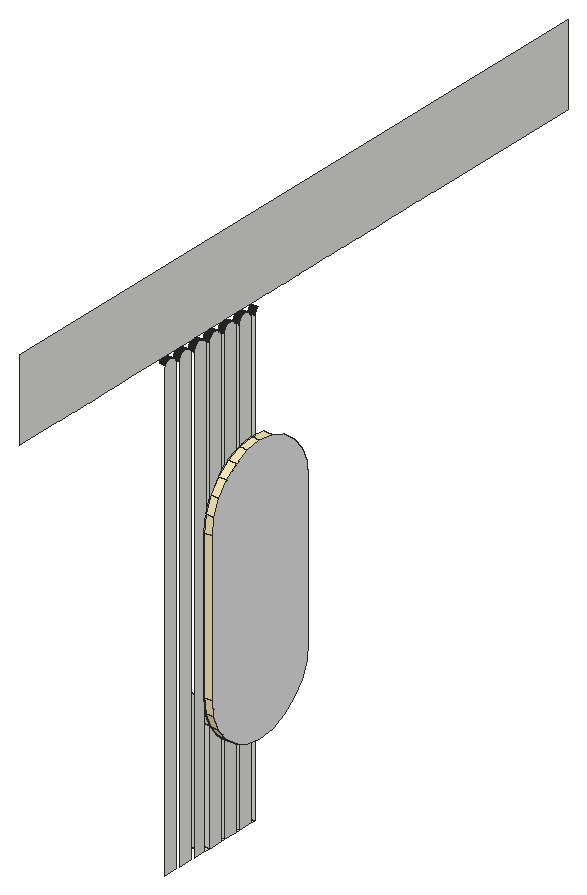
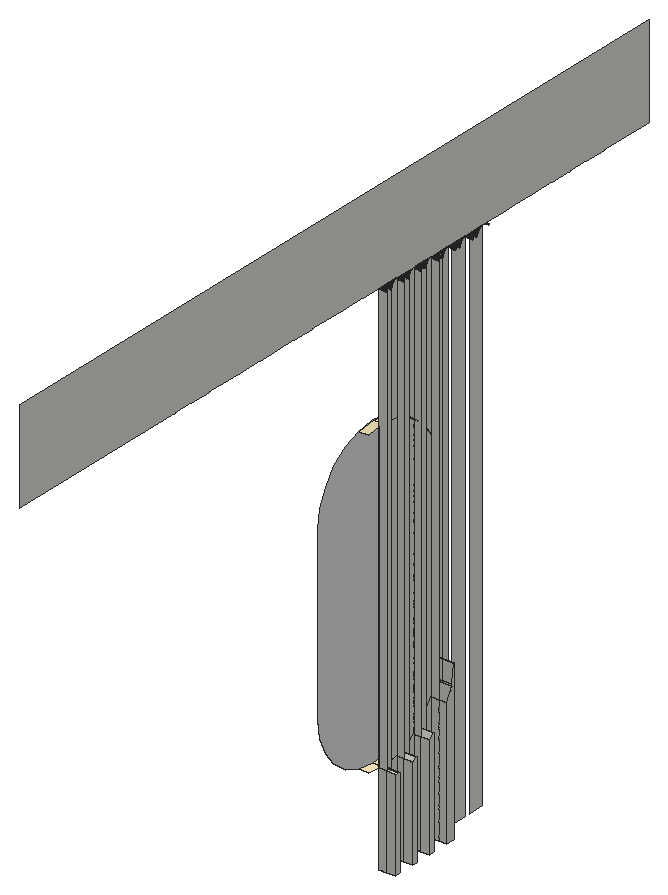
# SketchUp Ruby script. Lengths in inches.
U = 1.inch
M = Sketchup.active_model
def pt(a) = Geom::Point3d.new(a.map { |v| v * U })
def face(e, loops, mat)
  f = e.add_face(loops[0].map { |a| pt(a) })
  loops[1..].each { |l| e.add_face(l.map { |a| pt(a) }).erase! }
  f.material = f.back_material = mat if mat
  f
end
# faces: each face lists its corners as indices into pts; further lists are holes
def faces(e, pts, list, mat = nil) = list.each { |f| face(e, (f[0].is_a?(Array) ? f : [f]).map { |l| l.map { |i| pts[i] } }, mat) }
# xy, xz, yz: faces in a plane at the given z, y or x. An outline is a flat list of corners, or four numbers for a rectangle; further outlines are holes
def ring(l) = l.size == 4 ? [[l[0], l[1]], [l[2], l[1]], [l[2], l[3]], [l[0], l[3]]] : l.each_slice(2).to_a
def flat(e, list, mat, &to3) = list.each { |f| face(e, (f[0].is_a?(Array) ? f : [f]).map { |l| ring(l).map { |u, v| to3.(u, v) } }, mat) }
def xy(e, z, list, mat = nil) = flat(e, list, mat) { |x, y| [x, y, z] }
def xz(e, y, list, mat = nil) = flat(e, list, mat) { |x, z| [x, y, z] }
def yz(e, x, list, mat = nil) = flat(e, list, mat) { |y, z| [x, y, z] }
def lines(e, pts, list) = list.each { |a, b| e.add_line(pt(pts[a]), pt(pts[b])) }
# prism: a flat outline (further loops are holes) pulled along v
def prism(e, loops, v, mat = nil)
  f = face(e, loops, mat); d = Geom::Vector3d.new(v.map { |x| x * U })
  f.pushpull(f.normal.samedirection?(d) ? d.length : -d.length)
end
def box(e, o, s, mat = nil) = prism(e, [[o, [o[0] + s[0], o[1], o[2]], [o[0] + s[0], o[1] + s[1], o[2]], [o[0], o[1] + s[1], o[2]]]], [0, 0, s[2]], mat)
def at(x, y, z, deg = 0) = Geom::Transformation.translation(pt([x, y, z])) * Geom::Transformation.rotation(ORIGIN, Z_AXIS, deg.degrees)
def axes(o, x, y, z) = Geom::Transformation.new([*x, 0, *y, 0, *z, 0, *pt(o).to_a, 1])
def part(name) = M.definitions.add(name)
# library, detail: a bought-in or finely detailed component or shape, given as its bounding box
def library(name, o, s) = part(name).tap { |d| box(d.entities, o, s) }
def detail(e, o, s) = box(e.add_group.entities, o, s)
def put(e, d, t, mat = nil) = e.add_instance(d, t).tap { |i| i.material = mat if mat }
def group(e, t, mat = nil) = e.add_group.tap { |g| g.transformation = t; g.material = mat if mat }.entities
root = M.entities
M.materials.add("Heather_PantShadow").color = [249, 233, 187]
M.materials.add("[Mirror 02]").color = [229, 229, 229]
xy(root,39.466,[[7.875,42.018,10,43.106],[7.875,45.1875,10,45.893],[7.875,47.975,10,48.681],[7.875,50.762,10,51.468]])
xy(root,108,[[9,35.73,10,35.839],[9,38.517,10,38.626],[9,41.305,10,41.414],[9,44.092,10,44.201],[9,46.88,10,46.989],
  [9,49.667,10,49.776]])
xz(root,42.018,[[7.875,39.466,10,60.077]])
xz(root,42.018,[[10,60.077,11.25,82.153]],"Heather_PantShadow")
xz(root,43.106,[[7.875,39.466,9,55.879],[9,39.466,10,55.879],[9,55.879,10,106.961]])
xz(root,45.1875,[[7.875,39.466,9,53.349],[9,39.466,10,53.349],[9,53.349,10,106.961]])
xz(root,45.893,[[7.875,39.466,9,52.807],[9,39.466,10,52.807],[9,52.807,10,106.961]])
xz(root,47.975,[[7.875,39.466,9,51.741],[9,39.466,10,51.741],[9,51.741,10,106.961]])
xz(root,48.681,[[7.875,39.466,9,51.466],[9,39.466,10,51.466],[9,51.466,10,106.961]])
xz(root,50.762,[[7.875,39.466,9,51.192],[9,39.466,10,51.192],[9,51.192,10,106.961]])
xz(root,51.468,[[7.875,39.466,9,51.242],[9,39.466,10,51.242],[9,51.242,10,106.961]])
yz(root,7.875,[[42.018,39.466,43.106,39.466,43.106,55.879,42.4,57.583,42.322,57.772,42.018,60.077],[45.1875,39.466,45.893,39.466,45.893,52.807,45.1875,53.349],[47.975,39.466,48.681,39.466,48.681,51.466,48.62,51.474,47.975,51.741],[50.762,39.466,51.468,39.466,51.468,51.242,50.925,51.17,50.762,51.192]])
yz(root,9,[[9,108,16.217,108,16.272,108.001,16.326,108,19.005,108,19.059,108.001,19.114,108,21.792,108,21.847,108.001,21.901,108,24.58,108,24.634,108.001,24.689,108,27.367,108,27.422,108.001,27.476,108,30.155,108,30.209,108.001,30.264,108,32.942,108,32.997,108.001,33.051,108,35.73,108,35.784,108.001,35.839,108,38.517,108,38.572,108.001,38.626,108,41.305,108,41.359,108.001,41.414,108,44.092,108,44.147,108.001,44.201,108,46.88,108,46.934,108.001,46.989,108,49.667,108,49.722,108.001,49.776,108,52.455,108,52.509,108.001,52.564,108,55.242,108,55.297,108.001,55.351,108,58.03,108,58.084,108.001,58.139,108,60.817,108,60.872,108.001,60.926,108,63.605,108,63.659,108.001,63.714,108,66.392,108,66.447,108.001,66.501,108,69.18,108,69.234,108.001,69.289,108,71.967,108,72.022,108.001,72.076,108,74.755,108,74.809,108.001,74.864,108,77.542,108,77.597,108.001,77.651,108,80.33,108,80.384,108.001,80.439,108,83.117,108,83.172,108.001,83.226,108,85.905,108,85.959,108.001,86.014,108,111,108,111,120,9,120],[35.73,108,35.839,108,35.784,108.001],[38.517,108,38.626,108,38.572,108.001],[41.305,108,41.414,108,41.359,108.001],[44.092,108,44.201,108,44.147,108.001],
  [46.88,108,46.989,108,46.934,108.001],[49.667,108,49.776,108,49.722,108.001]])
yz(root,10,[[34.743,39.466,36.825,39.466,36.825,106.961,36.824,107.015,36.819,107.069,36.812,107.123,36.802,107.177,36.79,107.23,36.774,107.282,36.756,107.334,36.735,107.384,36.712,107.433,36.686,107.481,36.657,107.528,36.626,107.572,36.593,107.616,36.558,107.657,36.52,107.697,36.481,107.734,36.439,107.769,36.396,107.803,36.351,107.834,36.305,107.862,36.257,107.888,36.208,107.911,36.157,107.932,36.106,107.95,36.054,107.966,36.001,107.979,35.947,107.989,35.893,107.996,35.839,108,35.73,108,35.675,107.996,35.621,107.989,35.568,107.979,35.515,107.966,35.463,107.95,35.411,107.932,35.361,107.911,35.312,107.888,35.264,107.862,35.217,107.834,35.173,107.803,35.129,107.769,35.088,107.734,35.048,107.697,35.011,107.657,34.975,107.616,34.942,107.572,34.911,107.528,34.883,107.481,34.857,107.433,34.833,107.384,34.8125,107.334,34.794,107.282,34.779,107.23,34.766,107.177,34.756,107.123,34.749,107.069,34.745,107.015,34.743,106.961],[37.531,39.466,39.612,39.466,39.612,106.961,39.611,107.015,39.607,107.069,39.6,107.123,39.59,107.177,39.577,107.23,39.562,107.282,39.543,107.334,39.523,107.384,39.499,107.433,39.473,107.481,39.445,107.528,39.414,107.572,39.381,107.616,39.345,107.657,39.308,107.697,39.268,107.734,39.227,107.769,39.183,107.803,39.139,107.834,39.092,107.862,39.044,107.888,38.995,107.911,38.945,107.932,38.893,107.95,38.841,107.966,38.788,107.979,38.735,107.989,38.681,107.996,38.626,108,38.517,108,38.463,107.996,38.409,107.989,38.355,107.979,38.302,107.966,38.25,107.95,38.199,107.932,38.148,107.911,38.099,107.888,38.051,107.862,38.005,107.834,37.96,107.803,37.917,107.769,37.875,107.734,37.836,107.697,37.798,107.657,37.763,107.616,37.73,107.572,37.699,107.528,37.67,107.481,37.644,107.433,37.621,107.384,37.6,107.334,37.582,107.282,37.566,107.23,37.554,107.177,37.544,107.123,37.537,107.069,37.532,107.015,37.531,106.961],[40.318,39.466,42.018,39.466,42.018,82.153,42.322,84.458,42.4,84.647,42.4,106.961,42.399,107.015,42.394,107.069,42.387,107.123,42.377,107.177,42.365,107.23,42.349,107.282,42.331,107.334,42.31,107.384,42.287,107.433,42.261,107.481,42.232,107.528,42.201,107.572,42.168,107.616,42.133,107.657,42.095,107.697,42.056,107.734,42.014,107.769,41.971,107.803,41.926,107.834,41.88,107.862,41.832,107.888,41.783,107.911,41.732,107.932,41.681,107.95,41.629,107.966,41.576,107.979,41.522,107.989,41.468,107.996,41.414,108,41.305,108,41.25,107.996,41.196,107.989,41.143,107.979,41.09,107.966,41.038,107.95,40.986,107.932,40.936,107.911,40.887,107.888,40.839,107.862,40.792,107.834,40.748,107.803,40.704,107.769,40.663,107.734,40.623,107.697,40.586,107.657,40.55,107.616,40.517,107.572,40.486,107.528,40.458,107.481,40.432,107.433,40.408,107.384,40.388,107.334,40.369,107.282,40.354,107.23,40.341,107.177,40.331,107.123,40.324,107.069,40.32,107.015,40.318,106.961],[43.106,39.466,45.1875,39.466,45.1875,53.349,44.627,53.779,43.212,55.624,43.106,55.879],[45.893,39.466,47.975,39.466,47.975,51.741,46.472,52.364,45.893,52.807],
  [48.681,39.466,50.762,39.466,50.762,51.192,48.681,51.466],[50.925,51.17,50.762,51.192,50.762,91.038,50.925,91.06,51.468,90.988,51.468,51.242],[50.762,51.192,50.762,91.038,48.681,90.764,48.681,51.466],[48.681,51.466,48.62,51.474,47.975,51.741,47.975,90.489,48.62,90.756,48.681,90.764],[47.975,51.741,47.975,90.489,46.472,89.866,45.893,89.423,45.893,52.807,46.472,52.364],
  [45.893,52.807,45.1875,53.349,45.1875,88.881,45.893,89.423],[45.1875,53.349,45.1875,88.881,44.627,88.451,43.212,86.606,43.106,86.351,43.106,55.879,43.212,55.624,44.627,53.779],[43.106,55.879,42.4,57.583,42.4,84.647,43.106,86.351],[42.4,57.583,42.4,84.647,42.322,84.458,42.018,82.153,42.018,60.077,42.322,57.772],[43.106,86.351,43.212,86.606,44.627,88.451,45.1875,88.881,45.1875,106.961,45.186,107.015,45.182,107.069,45.175,107.123,45.165,107.177,45.152,107.23,45.137,107.282,45.118,107.334,45.098,107.384,45.074,107.433,45.048,107.481,45.02,107.528,44.989,107.572,44.956,107.616,44.92,107.657,44.883,107.697,44.843,107.734,44.802,107.769,44.758,107.803,44.714,107.834,44.667,107.862,44.619,107.888,44.57,107.911,44.52,107.932,44.468,107.95,44.416,107.966,44.363,107.979,44.31,107.989,44.256,107.996,44.201,108,44.092,108,44.038,107.996,43.984,107.989,43.93,107.979,43.877,107.966,43.825,107.95,43.774,107.932,43.723,107.911,43.674,107.888,43.626,107.862,43.58,107.834,43.535,107.803,43.492,107.769,43.45,107.734,43.411,107.697,43.373,107.657,43.338,107.616,43.305,107.572,43.274,107.528,43.245,107.481,43.219,107.433,43.196,107.384,43.175,107.334,43.157,107.282,43.141,107.23,43.129,107.177,43.119,107.123,43.112,107.069,43.107,107.015,43.106,106.961],
  [45.893,89.423,46.472,89.866,47.975,90.489,47.975,106.961,47.974,107.015,47.969,107.069,47.962,107.123,47.952,107.177,47.94,107.23,47.924,107.282,47.906,107.334,47.885,107.384,47.862,107.433,47.836,107.481,47.807,107.528,47.776,107.572,47.743,107.616,47.708,107.657,47.67,107.697,47.631,107.734,47.589,107.769,47.546,107.803,47.501,107.834,47.455,107.862,47.407,107.888,47.358,107.911,47.307,107.932,47.256,107.95,47.204,107.966,47.151,107.979,47.097,107.989,47.043,107.996,46.989,108,46.88,108,46.825,107.996,46.771,107.989,46.718,107.979,46.665,107.966,46.613,107.95,46.561,107.932,46.511,107.911,46.462,107.888,46.414,107.862,46.367,107.834,46.323,107.803,46.279,107.769,46.238,107.734,46.198,107.697,46.161,107.657,46.125,107.616,46.092,107.572,46.061,107.528,46.033,107.481,46.007,107.433,45.983,107.384,45.963,107.334,45.944,107.282,45.929,107.23,45.916,107.177,45.906,107.123,45.899,107.069,45.895,107.015,45.893,106.961],[48.681,90.764,50.762,91.038,50.762,106.961,50.761,107.015,50.757,107.069,50.75,107.123,50.74,107.177,50.727,107.23,50.712,107.282,50.693,107.334,50.673,107.384,50.649,107.433,50.623,107.481,50.595,107.528,50.564,107.572,50.531,107.616,50.495,107.657,50.458,107.697,50.418,107.734,50.377,107.769,50.333,107.803,50.289,107.834,50.242,107.862,50.194,107.888,50.145,107.911,50.095,107.932,50.043,107.95,49.991,107.966,49.938,107.979,49.885,107.989,49.831,107.996,49.776,108,49.667,108,49.613,107.996,49.559,107.989,49.505,107.979,49.452,107.966,49.4,107.95,49.349,107.932,49.298,107.911,49.249,107.888,49.201,107.862,49.155,107.834,49.11,107.803,49.067,107.769,49.025,107.734,48.986,107.697,48.948,107.657,48.913,107.616,48.88,107.572,48.849,107.528,48.82,107.481,48.794,107.433,48.771,107.384,48.75,107.334,48.732,107.282,48.716,107.23,48.704,107.177,48.694,107.123,48.687,107.069,48.682,107.015,48.681,106.961]])
yz(root,11.25,[[50.925,51.17,53.23,51.474,55.378,52.364,57.222,53.779,58.638,55.624,59.528,57.772,59.831,60.077,59.831,82.153,59.528,84.458,58.638,86.606,57.222,88.451,55.378,89.866,53.23,90.756,50.925,91.06,48.62,90.756,46.472,89.866,44.627,88.451,43.212,86.606,42.322,84.458,42.018,82.153,42.018,60.077,42.322,57.772,43.212,55.624,44.627,53.779,46.472,52.364,48.62,51.474]],"[Mirror 02]")
p = [[11.25,50.925,51.17],[11.25,48.62,51.474],[10,48.62,51.474],[10,48.681,51.466],[10,50.762,51.192],[10,50.925,51.17],
  [9,50.762,51.192],[7.875,50.762,51.192],[7.875,50.925,51.17],[10,51.468,51.242],[7.875,51.468,51.242],[9,51.468,51.242],
  [11.25,53.23,51.474],[10,53.23,51.474],[11.25,46.472,52.364],[10,46.472,52.364],[10,47.975,51.741],[9,47.975,51.741],
  [7.875,47.975,51.741],[7.875,48.62,51.474],[7.875,48.681,51.466],[9,48.681,51.466],[11.25,44.627,53.779],[10,44.627,53.779],
  [10,45.1875,53.349],[10,45.893,52.807],[9,45.1875,53.349],[7.875,45.1875,53.349],[7.875,45.893,52.807],[9,45.893,52.807],
  [11.25,43.212,55.624],[10,43.212,55.624],[11.25,42.322,57.772],[10,42.322,57.772],[10,42.4,57.583],[10,43.106,55.879],
  [9,42.4,57.583],[7.875,42.4,57.583],[7.875,43.106,55.879],[9,43.106,55.879],[7.875,42.322,57.772],[10,42.018,60.077],
  [7.875,42.018,60.077],[11.25,42.018,60.077],[11.25,42.018,82.153],[11.25,42.322,84.458],[10,42.322,84.458],[10,42.018,82.153],
  [11.25,43.212,86.606],[10,43.212,86.606],[10,43.106,86.351],[10,42.4,84.647],[11.25,44.627,88.451],[10,44.627,88.451],
  [11.25,46.472,89.866],[10,46.472,89.866],[10,45.893,89.423],[10,45.1875,88.881],[11.25,48.62,90.756],[10,48.62,90.756],
  [10,47.975,90.489],[11.25,50.925,91.06],[10,50.925,91.06],[10,50.762,91.038],[10,48.681,90.764],[11.25,53.23,90.756],
  [10,53.23,90.756],[10,51.468,90.988],[9,36.824,107.015],[9,36.819,107.069],[10,36.819,107.069],[10,36.824,107.015],
  [9,36.825,106.961],[10,36.825,106.961],[9,37.532,107.015],[9,37.531,106.961],[10,37.531,106.961],[10,37.532,107.015],
  [9,37.537,107.069],[10,37.537,107.069],[9,39.611,107.015],[9,39.607,107.069],[10,39.607,107.069],[10,39.611,107.015],
  [9,39.612,106.961],[10,39.612,106.961],[9,40.32,107.015],[9,40.318,106.961],[10,40.318,106.961],[10,40.32,107.015],
  [9,40.324,107.069],[10,40.324,107.069],[9,42.399,107.015],[9,42.394,107.069],[10,42.394,107.069],[10,42.399,107.015],
  [9,42.4,106.961],[10,42.4,106.961],[9,43.107,107.015],[9,43.106,106.961],[10,43.106,106.961],[10,43.107,107.015],
  [9,43.112,107.069],[10,43.112,107.069],[9,45.186,107.015],[9,45.182,107.069],[10,45.182,107.069],[10,45.186,107.015],
  [9,45.1875,106.961],[10,45.1875,106.961],[9,45.895,107.015],[9,45.893,106.961],[10,45.893,106.961],[10,45.895,107.015],
  [9,45.899,107.069],[10,45.899,107.069],[9,47.974,107.015],[9,47.969,107.069],[10,47.969,107.069],[10,47.974,107.015],
  [9,47.975,106.961],[10,47.975,106.961],[9,48.682,107.015],[9,48.681,106.961],[10,48.681,106.961],[10,48.682,107.015],
  [9,48.687,107.069],[10,48.687,107.069],[9,50.761,107.015],[9,50.757,107.069],[10,50.757,107.069],[10,50.761,107.015],
  [9,50.762,106.961],[10,50.762,106.961],[9,51.47,107.015],[9,51.468,106.961],[10,51.468,106.961],[10,51.47,107.015],
  [9,51.474,107.069],[10,51.474,107.069],[9,36.812,107.123],[9,36.802,107.177],[10,36.802,107.177],[10,36.812,107.123],
  [9,37.544,107.123],[10,37.544,107.123],[9,37.554,107.177],[10,37.554,107.177],[9,39.6,107.123],[9,39.59,107.177],
  [10,39.59,107.177],[10,39.6,107.123],[9,40.331,107.123],[10,40.331,107.123],[9,40.341,107.177],[10,40.341,107.177],
  [9,42.387,107.123],[9,42.377,107.177],[10,42.377,107.177],[10,42.387,107.123],[9,43.119,107.123],[10,43.119,107.123],
  [9,43.129,107.177],[10,43.129,107.177],[9,45.175,107.123],[9,45.165,107.177],[10,45.165,107.177],[10,45.175,107.123],
  [9,45.906,107.123],[10,45.906,107.123],[9,45.916,107.177],[10,45.916,107.177],[9,47.962,107.123],[9,47.952,107.177],
  [10,47.952,107.177],[10,47.962,107.123],[9,48.694,107.123],[10,48.694,107.123],[9,48.704,107.177],[10,48.704,107.177],
  [9,50.75,107.123],[9,50.74,107.177],[10,50.74,107.177],[10,50.75,107.123],[9,51.481,107.123],[10,51.481,107.123],
  [9,51.491,107.177],[10,51.491,107.177],[9,36.79,107.23],[9,36.774,107.282],[10,36.774,107.282],[10,36.79,107.23],
  [9,37.566,107.23],[10,37.566,107.23],[9,37.582,107.282],[10,37.582,107.282],[9,39.577,107.23],[9,39.562,107.282],
  [10,39.562,107.282],[10,39.577,107.23],[9,40.354,107.23],[10,40.354,107.23],[9,40.369,107.282],[10,40.369,107.282],
  [9,42.365,107.23],[9,42.349,107.282],[10,42.349,107.282],[10,42.365,107.23],[9,43.141,107.23],[10,43.141,107.23],
  [9,43.157,107.282],[10,43.157,107.282],[9,45.152,107.23],[9,45.137,107.282],[10,45.137,107.282],[10,45.152,107.23],
  [9,45.929,107.23],[10,45.929,107.23],[9,45.944,107.282],[10,45.944,107.282],[9,47.94,107.23],[9,47.924,107.282],
  [10,47.924,107.282],[10,47.94,107.23],[9,48.716,107.23],[10,48.716,107.23],[9,48.732,107.282],[10,48.732,107.282],
  [9,50.727,107.23],[9,50.712,107.282],[10,50.712,107.282],[10,50.727,107.23],[9,51.504,107.23],[10,51.504,107.23],
  [9,51.519,107.282],[10,51.519,107.282],[9,36.756,107.334],[9,36.735,107.384],[10,36.735,107.384],[10,36.756,107.334],
  [9,37.6,107.334],[10,37.6,107.334],[9,37.621,107.384],[10,37.621,107.384],[9,39.543,107.334],[9,39.523,107.384],
  [10,39.523,107.384],[10,39.543,107.334],[9,40.388,107.334],[10,40.388,107.334],[9,40.408,107.384],[10,40.408,107.384],
  [9,42.331,107.334],[9,42.31,107.384],[10,42.31,107.384],[10,42.331,107.334],[9,43.175,107.334],[10,43.175,107.334],
  [9,43.196,107.384],[10,43.196,107.384],[9,45.118,107.334],[9,45.098,107.384],[10,45.098,107.384],[10,45.118,107.334],
  [9,45.963,107.334],[10,45.963,107.334],[9,45.983,107.384],[10,45.983,107.384],[9,47.906,107.334],[9,47.885,107.384],
  [10,47.885,107.384],[10,47.906,107.334],[9,48.75,107.334],[10,48.75,107.334],[9,48.771,107.384],[10,48.771,107.384],
  [9,50.693,107.334],[9,50.673,107.384],[10,50.673,107.384],[10,50.693,107.334],[9,51.538,107.334],[10,51.538,107.334],
  [9,51.558,107.384],[10,51.558,107.384],[9,36.712,107.433],[9,36.686,107.481],[10,36.686,107.481],[10,36.712,107.433],
  [9,37.644,107.433],[10,37.644,107.433],[9,37.67,107.481],[10,37.67,107.481],[9,39.499,107.433],[9,39.473,107.481],
  [10,39.473,107.481],[10,39.499,107.433],[9,40.432,107.433],[10,40.432,107.433],[9,40.458,107.481],[10,40.458,107.481],
  [9,42.287,107.433],[9,42.261,107.481],[10,42.261,107.481],[10,42.287,107.433],[9,43.219,107.433],[10,43.219,107.433],
  [9,43.245,107.481],[10,43.245,107.481],[9,45.074,107.433],[9,45.048,107.481],[10,45.048,107.481],[10,45.074,107.433],
  [9,46.007,107.433],[10,46.007,107.433],[9,46.033,107.481],[10,46.033,107.481],[9,47.862,107.433],[9,47.836,107.481],
  [10,47.836,107.481],[10,47.862,107.433],[9,48.794,107.433],[10,48.794,107.433],[9,48.82,107.481],[10,48.82,107.481],
  [9,50.649,107.433],[9,50.623,107.481],[10,50.623,107.481],[10,50.649,107.433],[9,51.582,107.433],[10,51.582,107.433],
  [9,51.608,107.481],[10,51.608,107.481],[9,36.657,107.528],[9,36.626,107.572],[10,36.626,107.572],[10,36.657,107.528],
  [9,37.699,107.528],[10,37.699,107.528],[9,37.73,107.572],[10,37.73,107.572],[9,39.445,107.528],[9,39.414,107.572],
  [10,39.414,107.572],[10,39.445,107.528],[9,40.486,107.528],[10,40.486,107.528],[9,40.517,107.572],[10,40.517,107.572],
  [9,42.232,107.528],[9,42.201,107.572],[10,42.201,107.572],[10,42.232,107.528],[9,43.274,107.528],[10,43.274,107.528],
  [9,43.305,107.572],[10,43.305,107.572],[9,45.02,107.528],[9,44.989,107.572],[10,44.989,107.572],[10,45.02,107.528],
  [9,46.061,107.528],[10,46.061,107.528],[9,46.092,107.572],[10,46.092,107.572],[9,47.807,107.528],[9,47.776,107.572],
  [10,47.776,107.572],[10,47.807,107.528],[9,48.849,107.528],[10,48.849,107.528],[9,48.88,107.572],[10,48.88,107.572],
  [9,50.595,107.528],[9,50.564,107.572],[10,50.564,107.572],[10,50.595,107.528],[9,51.636,107.528],[10,51.636,107.528],
  [9,51.667,107.572],[10,51.667,107.572],[9,34.975,107.616],[9,34.942,107.572],[10,34.942,107.572],[10,34.975,107.616],
  [9,35.011,107.657],[10,35.011,107.657],[9,36.593,107.616],[9,36.558,107.657],[10,36.558,107.657],[10,36.593,107.616],
  [9,37.763,107.616],[10,37.763,107.616],[9,37.798,107.657],[10,37.798,107.657],[9,39.381,107.616],[9,39.345,107.657],
  [10,39.345,107.657],[10,39.381,107.616],[9,40.55,107.616],[10,40.55,107.616],[9,40.586,107.657],[10,40.586,107.657],
  [9,42.168,107.616],[9,42.133,107.657],[10,42.133,107.657],[10,42.168,107.616],[9,43.338,107.616],[10,43.338,107.616],
  [9,43.373,107.657],[10,43.373,107.657],[9,44.956,107.616],[9,44.92,107.657],[10,44.92,107.657],[10,44.956,107.616],
  [9,46.125,107.616],[10,46.125,107.616],[9,46.161,107.657],[10,46.161,107.657],[9,47.743,107.616],[9,47.708,107.657],
  [10,47.708,107.657],[10,47.743,107.616],[9,48.913,107.616],[10,48.913,107.616],[9,48.948,107.657],[10,48.948,107.657],
  [9,50.531,107.616],[9,50.495,107.657],[10,50.495,107.657],[10,50.531,107.616],[9,51.7,107.616],[10,51.7,107.616],
  [9,51.736,107.657],[10,51.736,107.657],[9,35.048,107.697],[10,35.048,107.697],[9,35.088,107.734],[10,35.088,107.734],
  [9,35.129,107.769],[10,35.129,107.769],[9,36.481,107.734],[9,36.439,107.769],[10,36.439,107.769],[10,36.481,107.734],
  [9,36.52,107.697],[10,36.52,107.697],[9,37.836,107.697],[10,37.836,107.697],[9,37.875,107.734],[10,37.875,107.734],
  [9,37.917,107.769],[10,37.917,107.769],[9,39.268,107.734],[9,39.227,107.769],[10,39.227,107.769],[10,39.268,107.734],
  [9,39.308,107.697],[10,39.308,107.697],[9,40.623,107.697],[10,40.623,107.697],[9,40.663,107.734],[10,40.663,107.734],
  [9,40.704,107.769],[10,40.704,107.769],[9,42.056,107.734],[9,42.014,107.769],[10,42.014,107.769],[10,42.056,107.734],
  [9,42.095,107.697],[10,42.095,107.697],[9,43.411,107.697],[10,43.411,107.697],[9,43.45,107.734],[10,43.45,107.734],
  [9,43.492,107.769],[10,43.492,107.769],[9,44.843,107.734],[9,44.802,107.769],[10,44.802,107.769],[10,44.843,107.734],
  [9,44.883,107.697],[10,44.883,107.697],[9,46.198,107.697],[10,46.198,107.697],[9,46.238,107.734],[10,46.238,107.734],
  [9,46.279,107.769],[10,46.279,107.769],[9,47.631,107.734],[9,47.589,107.769],[10,47.589,107.769],[10,47.631,107.734],
  [9,47.67,107.697],[10,47.67,107.697],[9,48.986,107.697],[10,48.986,107.697],[9,49.025,107.734],[10,49.025,107.734],
  [9,49.067,107.769],[10,49.067,107.769],[9,50.418,107.734],[9,50.377,107.769],[10,50.377,107.769],[10,50.418,107.734],
  [9,50.458,107.697],[10,50.458,107.697],[9,51.773,107.697],[10,51.773,107.697],[9,51.813,107.734],[10,51.813,107.734],
  [9,51.854,107.769],[10,51.854,107.769],[9,35.173,107.803],[10,35.173,107.803],[9,35.217,107.834],[10,35.217,107.834],
  [9,35.264,107.862],[10,35.264,107.862],[9,36.351,107.834],[9,36.305,107.862],[10,36.305,107.862],[10,36.351,107.834],
  [9,36.396,107.803],[10,36.396,107.803],[9,37.96,107.803],[10,37.96,107.803],[9,38.005,107.834],[10,38.005,107.834],
  [9,38.051,107.862],[10,38.051,107.862],[9,39.139,107.834],[9,39.092,107.862],[10,39.092,107.862],[10,39.139,107.834],
  [9,39.183,107.803],[10,39.183,107.803],[9,40.748,107.803],[10,40.748,107.803],[9,40.792,107.834],[10,40.792,107.834],
  [9,40.839,107.862],[10,40.839,107.862],[9,41.926,107.834],[9,41.88,107.862],[10,41.88,107.862],[10,41.926,107.834],
  [9,41.971,107.803],[10,41.971,107.803],[9,43.535,107.803],[10,43.535,107.803],[9,43.58,107.834],[10,43.58,107.834],
  [9,43.626,107.862],[10,43.626,107.862],[9,44.714,107.834],[9,44.667,107.862],[10,44.667,107.862],[10,44.714,107.834],
  [9,44.758,107.803],[10,44.758,107.803],[9,46.323,107.803],[10,46.323,107.803],[9,46.367,107.834],[10,46.367,107.834],
  [9,46.414,107.862],[10,46.414,107.862],[9,47.501,107.834],[9,47.455,107.862],[10,47.455,107.862],[10,47.501,107.834],
  [9,47.546,107.803],[10,47.546,107.803],[9,49.11,107.803],[10,49.11,107.803],[9,49.155,107.834],[10,49.155,107.834],
  [9,49.201,107.862],[10,49.201,107.862],[9,50.289,107.834],[9,50.242,107.862],[10,50.242,107.862],[10,50.289,107.834],
  [9,50.333,107.803],[10,50.333,107.803],[9,51.898,107.803],[10,51.898,107.803],[9,51.942,107.834],[10,51.942,107.834],
  [9,51.989,107.862],[10,51.989,107.862],[9,35.312,107.888],[10,35.312,107.888],[9,35.361,107.911],[10,35.361,107.911],
  [9,35.411,107.932],[10,35.411,107.932],[9,35.463,107.95],[10,35.463,107.95],[9,36.157,107.932],[9,36.106,107.95],
  [10,36.106,107.95],[10,36.157,107.932],[9,36.208,107.911],[10,36.208,107.911],[9,36.257,107.888],[10,36.257,107.888],
  [9,38.099,107.888],[10,38.099,107.888],[9,38.148,107.911],[10,38.148,107.911],[9,38.199,107.932],[10,38.199,107.932],
  [9,38.25,107.95],[10,38.25,107.95],[9,38.945,107.932],[9,38.893,107.95],[10,38.893,107.95],[10,38.945,107.932],
  [9,38.995,107.911],[10,38.995,107.911],[9,39.044,107.888],[10,39.044,107.888],[9,40.887,107.888],[10,40.887,107.888],
  [9,40.936,107.911],[10,40.936,107.911],[9,40.986,107.932],[10,40.986,107.932],[9,41.038,107.95],[10,41.038,107.95],
  [9,41.732,107.932],[9,41.681,107.95],[10,41.681,107.95],[10,41.732,107.932],[9,41.783,107.911],[10,41.783,107.911],
  [9,41.832,107.888],[10,41.832,107.888],[9,43.674,107.888],[10,43.674,107.888],[9,43.723,107.911],[10,43.723,107.911],
  [9,43.774,107.932],[10,43.774,107.932],[9,43.825,107.95],[10,43.825,107.95],[9,44.52,107.932],[9,44.468,107.95],
  [10,44.468,107.95],[10,44.52,107.932],[9,44.57,107.911],[10,44.57,107.911],[9,44.619,107.888],[10,44.619,107.888],
  [9,46.462,107.888],[10,46.462,107.888],[9,46.511,107.911],[10,46.511,107.911],[9,46.561,107.932],[10,46.561,107.932],
  [9,46.613,107.95],[10,46.613,107.95],[9,47.307,107.932],[9,47.256,107.95],[10,47.256,107.95],[10,47.307,107.932],
  [9,47.358,107.911],[10,47.358,107.911],[9,47.407,107.888],[10,47.407,107.888],[9,49.249,107.888],[10,49.249,107.888],
  [9,49.298,107.911],[10,49.298,107.911],[9,49.349,107.932],[10,49.349,107.932],[9,49.4,107.95],[10,49.4,107.95],
  [9,50.095,107.932],[9,50.043,107.95],[10,50.043,107.95],[10,50.095,107.932],[9,50.145,107.911],[10,50.145,107.911],
  [9,50.194,107.888],[10,50.194,107.888],[9,52.037,107.888],[10,52.037,107.888],[9,35.515,107.966],[10,35.515,107.966],
  [9,35.568,107.979],[10,35.568,107.979],[9,35.621,107.989],[10,35.621,107.989],[9,35.675,107.996],[10,35.675,107.996],
  [9,35.73,108],[10,35.73,108],[9,35.893,107.996],[9,35.839,108],[10,35.839,108],[10,35.893,107.996],
  [9,35.947,107.989],[10,35.947,107.989],[9,36.001,107.979],[10,36.001,107.979],[9,36.054,107.966],[10,36.054,107.966],
  [9,38.302,107.966],[10,38.302,107.966],[9,38.355,107.979],[10,38.355,107.979],[9,38.409,107.989],[10,38.409,107.989],
  [9,38.463,107.996],[10,38.463,107.996],[9,38.517,108],[10,38.517,108],[9,38.681,107.996],[9,38.626,108],
  [10,38.626,108],[10,38.681,107.996],[9,38.735,107.989],[10,38.735,107.989],[9,38.788,107.979],[10,38.788,107.979],
  [9,38.841,107.966],[10,38.841,107.966],[9,41.09,107.966],[10,41.09,107.966],[9,41.143,107.979],[10,41.143,107.979],
  [9,41.196,107.989],[10,41.196,107.989],[9,41.25,107.996],[10,41.25,107.996],[9,41.305,108],[10,41.305,108],
  [9,41.468,107.996],[9,41.414,108],[10,41.414,108],[10,41.468,107.996],[9,41.522,107.989],[10,41.522,107.989],
  [9,41.576,107.979],[10,41.576,107.979],[9,41.629,107.966],[10,41.629,107.966],[9,43.877,107.966],[10,43.877,107.966],
  [9,43.93,107.979],[10,43.93,107.979],[9,43.984,107.989],[10,43.984,107.989],[9,44.038,107.996],[10,44.038,107.996],
  [9,44.092,108],[10,44.092,108],[9,44.256,107.996],[9,44.201,108],[10,44.201,108],[10,44.256,107.996],
  [9,44.31,107.989],[10,44.31,107.989],[9,44.363,107.979],[10,44.363,107.979],[9,44.416,107.966],[10,44.416,107.966],
  [9,46.665,107.966],[10,46.665,107.966],[9,46.718,107.979],[10,46.718,107.979],[9,46.771,107.989],[10,46.771,107.989],
  [9,46.825,107.996],[10,46.825,107.996],[9,46.88,108],[10,46.88,108],[9,47.043,107.996],[9,46.989,108],
  [10,46.989,108],[10,47.043,107.996],[9,47.097,107.989],[10,47.097,107.989],[9,47.151,107.979],[10,47.151,107.979],
  [9,47.204,107.966],[10,47.204,107.966],[9,49.452,107.966],[10,49.452,107.966],[9,49.505,107.979],[10,49.505,107.979],
  [9,49.559,107.989],[10,49.559,107.989],[9,49.613,107.996],[10,49.613,107.996],[9,49.667,108],[10,49.667,108],
  [9,49.831,107.996],[9,49.776,108],[10,49.776,108],[10,49.831,107.996],[9,49.885,107.989],[10,49.885,107.989],
  [9,49.938,107.979],[10,49.938,107.979],[9,49.991,107.966],[10,49.991,107.966],[9,42.4,39.466],[7.875,42.4,39.466]]
faces(root,p,[[0,1,2,3,4,5],[12,0,5,9,13],[1,14,15,16,2],[14,22,23,24,25,15],[22,30,31,23],[30,32,33,34,35,31],[32,43,41,33],[44,45,46,47],
  [45,48,49,50,51,46],[48,52,53,49],[52,54,55,56,57,53],[54,58,59,60,55],[58,61,62,63,64,59],[61,65,66,67,62]],"Heather_PantShadow")
faces(root,p,[[5,4,6,7,8],[9,5,8,10,11],[2,16,17,18,19],[3,2,19,20,21],[25,24,26,27,28,29],[35,34,36,37,38,39],[34,33,40,37,36],[33,41,42,40],
  [68,69,70,71],[72,68,71,73],[74,75,76,77],[78,74,77,79],[80,81,82,83],[84,80,83,85],[86,87,88,89],[90,86,89,91],
  [92,93,94,95],[96,92,95,97],[98,99,100,101],[102,98,101,103],[104,105,106,107],[108,104,107,109],[110,111,112,113],[114,110,113,115],
  [116,117,118,119],[120,116,119,121],[122,123,124,125],[126,122,125,127],[128,129,130,131],[132,128,131,133],[134,135,136,137],[138,134,137,139],
  [140,141,142,143],[69,140,143,70],[144,78,79,145],[146,144,145,147],[148,149,150,151],[81,148,151,82],[152,90,91,153],[154,152,153,155],
  [156,157,158,159],[93,156,159,94],[160,102,103,161],[162,160,161,163],[164,165,166,167],[105,164,167,106],[168,114,115,169],[170,168,169,171],
  [172,173,174,175],[117,172,175,118],[176,126,127,177],[178,176,177,179],[180,181,182,183],[129,180,183,130],[184,138,139,185],[186,184,185,187],
  [188,189,190,191],[141,188,191,142],[192,146,147,193],[194,192,193,195],[196,197,198,199],[149,196,199,150],[200,154,155,201],[202,200,201,203],
  [204,205,206,207],[157,204,207,158],[208,162,163,209],[210,208,209,211],[212,213,214,215],[165,212,215,166],[216,170,171,217],[218,216,217,219],
  [220,221,222,223],[173,220,223,174],[224,178,179,225],[226,224,225,227],[228,229,230,231],[181,228,231,182],[232,186,187,233],[234,232,233,235],
  [236,237,238,239],[189,236,239,190],[240,194,195,241],[242,240,241,243],[244,245,246,247],[197,244,247,198],[248,202,203,249],[250,248,249,251],
  [252,253,254,255],[205,252,255,206],[256,210,211,257],[258,256,257,259],[260,261,262,263],[213,260,263,214],[264,218,219,265],[266,264,265,267],
  [268,269,270,271],[221,268,271,222],[272,226,227,273],[274,272,273,275],[276,277,278,279],[229,276,279,230],[280,234,235,281],[282,280,281,283],
  [284,285,286,287],[237,284,287,238],[288,242,243,289],[290,288,289,291],[292,293,294,295],[245,292,295,246],[296,250,251,297],[298,296,297,299],
  [300,301,302,303],[253,300,303,254],[304,258,259,305],[306,304,305,307],[308,309,310,311],[261,308,311,262],[312,266,267,313],[314,312,313,315],
  [316,317,318,319],[269,316,319,270],[320,274,275,321],[322,320,321,323],[324,325,326,327],[277,324,327,278],[328,282,283,329],[330,328,329,331],
  [332,333,334,335],[285,332,335,286],[336,290,291,337],[338,336,337,339],[340,341,342,343],[293,340,343,294],[344,298,299,345],[346,344,345,347],
  [348,349,350,351],[301,348,351,302],[352,306,307,353],[354,352,353,355],[356,357,358,359],[309,356,359,310],[360,314,315,361],[362,360,361,363],
  [364,365,366,367],[317,364,367,318],[368,322,323,369],[370,368,369,371],[372,373,374,375],[325,372,375,326],[376,330,331,377],[378,376,377,379],
  [380,381,382,383],[384,380,383,385],[386,387,388,389],[333,386,389,334],[390,338,339,391],[392,390,391,393],[394,395,396,397],[341,394,397,342],
  [398,346,347,399],[400,398,399,401],[402,403,404,405],[349,402,405,350],[406,354,355,407],[408,406,407,409],[410,411,412,413],[357,410,413,358],
  [414,362,363,415],[416,414,415,417],[418,419,420,421],[365,418,421,366],[422,370,371,423],[424,422,423,425],[426,427,428,429],[373,426,429,374],
  [430,378,379,431],[432,430,431,433],[434,384,385,435],[436,434,435,437],[438,436,437,439],[440,441,442,443],[444,440,443,445],[387,444,445,388],
  [446,392,393,447],[448,446,447,449],[450,448,449,451],[452,453,454,455],[456,452,455,457],[395,456,457,396],[458,400,401,459],[460,458,459,461],
  [462,460,461,463],[464,465,466,467],[468,464,467,469],[403,468,469,404],[470,408,409,471],[472,470,471,473],[474,472,473,475],[476,477,478,479],
  [480,476,479,481],[411,480,481,412],[482,416,417,483],[484,482,483,485],[486,484,485,487],[488,489,490,491],[492,488,491,493],[419,492,493,420],
  [494,424,425,495],[496,494,495,497],[498,496,497,499],[500,501,502,503],[504,500,503,505],[427,504,505,428],[506,432,433,507],[508,506,507,509],
  [510,508,509,511],[512,438,439,513],[514,512,513,515],[516,514,515,517],[518,519,520,521],[522,518,521,523],[441,522,523,442],[524,450,451,525],
  [526,524,525,527],[528,526,527,529],[530,531,532,533],[534,530,533,535],[453,534,535,454],[536,462,463,537],[538,536,537,539],[540,538,539,541],
  [542,543,544,545],[546,542,545,547],[465,546,547,466],[548,474,475,549],[550,548,549,551],[552,550,551,553],[554,555,556,557],[558,554,557,559],
  [477,558,559,478],[560,486,487,561],[562,560,561,563],[564,562,563,565],[566,567,568,569],[570,566,569,571],[489,570,571,490],[572,498,499,573],
  [574,572,573,575],[576,574,575,577],[578,579,580,581],[582,578,581,583],[501,582,583,502],[584,510,511,585],[586,584,585,587],[588,586,587,589],
  [590,516,517,591],[592,590,591,593],[594,592,593,595],[596,594,595,597],[598,599,600,601],[602,598,601,603],[604,602,603,605],[519,604,605,520],
  [606,528,529,607],[608,606,607,609],[610,608,609,611],[612,610,611,613],[614,615,616,617],[618,614,617,619],[620,618,619,621],[531,620,621,532],
  [622,540,541,623],[624,622,623,625],[626,624,625,627],[628,626,627,629],[630,631,632,633],[634,630,633,635],[636,634,635,637],[543,636,637,544],
  [638,552,553,639],[640,638,639,641],[642,640,641,643],[644,642,643,645],[646,647,648,649],[650,646,649,651],[652,650,651,653],[555,652,653,556],
  [654,564,565,655],[656,654,655,657],[658,656,657,659],[660,658,659,661],[662,663,664,665],[666,662,665,667],[668,666,667,669],[567,668,669,568],
  [670,576,577,671],[672,670,671,673],[674,672,673,675],[676,674,675,677],[678,679,680,681],[682,678,681,683],[684,682,683,685],[579,684,685,580],
  [686,588,589,687],[688,596,597,689],[690,688,689,691],[692,690,691,693],[694,692,693,695],[696,694,695,697],[698,699,700,701],[702,698,701,703],
  [704,702,703,705],[706,704,705,707],[599,706,707,600],[708,612,613,709],[710,708,709,711],[712,710,711,713],[714,712,713,715],[716,714,715,717],
  [718,719,720,721],[722,718,721,723],[724,722,723,725],[726,724,725,727],[615,726,727,616],[728,628,629,729],[730,728,729,731],[732,730,731,733],
  [734,732,733,735],[736,734,735,737],[738,739,740,741],[742,738,741,743],[744,742,743,745],[746,744,745,747],[631,746,747,632],[748,644,645,749],
  [750,748,749,751],[752,750,751,753],[754,752,753,755],[756,754,755,757],[758,759,760,761],[762,758,761,763],[764,762,763,765],[766,764,765,767],
  [647,766,767,648],[768,660,661,769],[770,768,769,771],[772,770,771,773],[774,772,773,775],[776,774,775,777],[778,779,780,781],[782,778,781,783],
  [784,782,783,785],[786,784,785,787],[663,786,787,664],[788,676,677,789],[790,788,789,791],[792,790,791,793],[794,792,793,795],[796,794,795,797],
  [798,799,800,801],[802,798,801,803],[804,802,803,805],[806,804,805,807],[679,806,807,680]])
lines(root,p,[[36,96],[808,809]])
